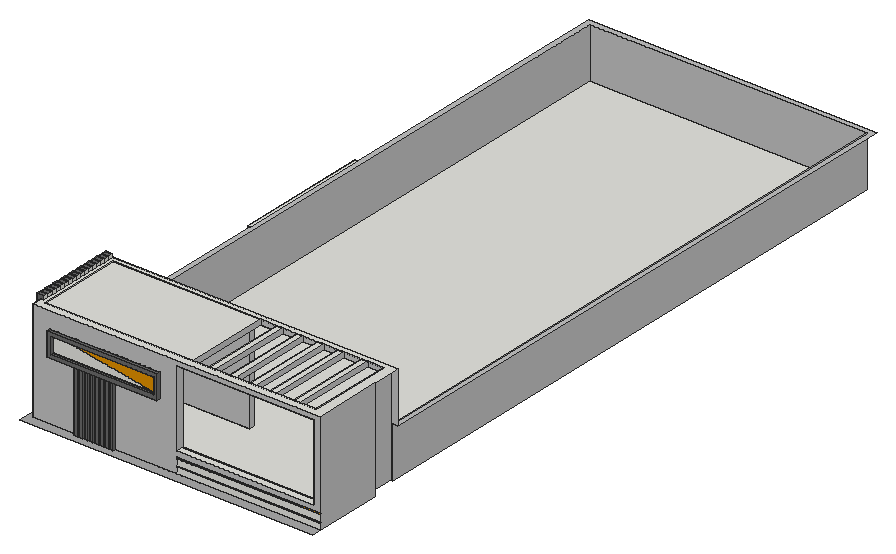
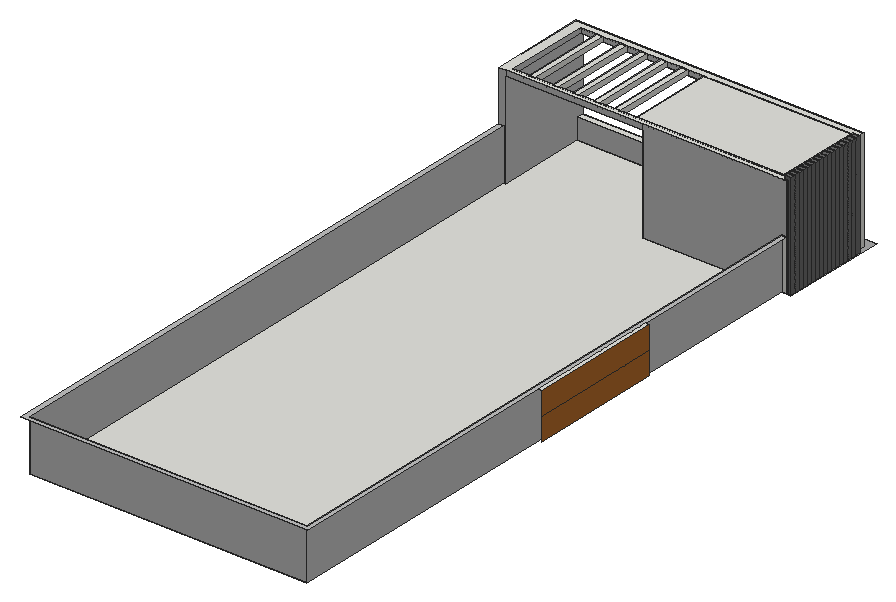
# SketchUp Ruby script. Lengths in inches.
U = 1.inch
M = Sketchup.active_model
def pt(a) = Geom::Point3d.new(a.map { |v| v * U })
def face(e, loops, mat)
  f = e.add_face(loops[0].map { |a| pt(a) })
  loops[1..].each { |l| e.add_face(l.map { |a| pt(a) }).erase! }
  f.material = f.back_material = mat if mat
  f
end
# faces: each face lists its corners as indices into pts; further lists are holes
def faces(e, pts, list, mat = nil) = list.each { |f| face(e, (f[0].is_a?(Array) ? f : [f]).map { |l| l.map { |i| pts[i] } }, mat) }
# xy, xz, yz: faces in a plane at the given z, y or x. An outline is a flat list of corners, or four numbers for a rectangle; further outlines are holes
def ring(l) = l.size == 4 ? [[l[0], l[1]], [l[2], l[1]], [l[2], l[3]], [l[0], l[3]]] : l.each_slice(2).to_a
def flat(e, list, mat, &to3) = list.each { |f| face(e, (f[0].is_a?(Array) ? f : [f]).map { |l| ring(l).map { |u, v| to3.(u, v) } }, mat) }
def xy(e, z, list, mat = nil) = flat(e, list, mat) { |x, y| [x, y, z] }
def xz(e, y, list, mat = nil) = flat(e, list, mat) { |x, z| [x, y, z] }
def yz(e, x, list, mat = nil) = flat(e, list, mat) { |y, z| [x, y, z] }
def lines(e, pts, list) = list.each { |a, b| e.add_line(pt(pts[a]), pt(pts[b])) }
# prism: a flat outline (further loops are holes) pulled along v
def prism(e, loops, v, mat = nil)
  f = face(e, loops, mat); d = Geom::Vector3d.new(v.map { |x| x * U })
  f.pushpull(f.normal.samedirection?(d) ? d.length : -d.length)
end
def box(e, o, s, mat = nil) = prism(e, [[o, [o[0] + s[0], o[1], o[2]], [o[0] + s[0], o[1] + s[1], o[2]], [o[0], o[1] + s[1], o[2]]]], [0, 0, s[2]], mat)
def at(x, y, z, deg = 0) = Geom::Transformation.translation(pt([x, y, z])) * Geom::Transformation.rotation(ORIGIN, Z_AXIS, deg.degrees)
def axes(o, x, y, z) = Geom::Transformation.new([*x, 0, *y, 0, *z, 0, *pt(o).to_a, 1])
def part(name) = M.definitions.add(name)
# library, detail: a bought-in or finely detailed component or shape, given as its bounding box
def library(name, o, s) = part(name).tap { |d| box(d.entities, o, s) }
def detail(e, o, s) = box(e.add_group.entities, o, s)
def put(e, d, t, mat = nil) = e.add_instance(d, t).tap { |i| i.material = mat if mat }
def group(e, t, mat = nil) = e.add_group.tap { |g| g.transformation = t; g.material = mat if mat }.entities
root = M.entities
M.materials.add("[0038_Orange]").color = [221, 143, 0]
M.materials.add("[0131_Silver]").color = [192, 192, 192]
M.materials.add("[0132_LightGray]").color = [169, 169, 169]
M.materials.add("[0134_DimGray]").color = [105, 105, 105]
M.materials.add("[Wood Bamboo]").color = [177, 105, 43]
xy(root,996,[[72,36,72,378,582,378,582,360,96,360,96,60,582,60,582,36],[582,36,1068,60],[96,60,1068,60,1068,378,1074,378,1074,2478,90,2478,90,378,582,378,582,360,96,360],[57.95,71.51,70.26,86.51],[57.95,89.51,70.26,104.51],
  [57.95,107.51,70.26,122.51],[57.95,125.51,70.26,140.51],[57.95,143.51,70.26,158.51],[57.95,161.51,70.26,176.51],[57.95,179.51,70.26,194.51],
  [57.95,197.51,70.26,212.51],[57.95,215.51,70.26,230.51],[57.95,233.51,70.26,248.51],[57.95,251.51,70.26,266.51],[57.95,269.51,70.26,284.51],
  [57.95,287.51,70.26,302.51],[57.95,305.51,70.26,320.51],[57.95,323.51,70.26,338.51],[57.95,341.51,70.26,356.51],[57.95,359.51,70.26,374.51]])
xy(root,996,[[[56,0,1092,0,1092,36,72,36,72,378,56,378],[57.95,359.51,70.26,374.51],[57.95,341.51,70.26,356.51],[57.95,323.51,70.26,338.51],[57.95,305.51,70.26,320.51],[57.95,287.51,70.26,302.51],[57.95,269.51,70.26,284.51],[57.95,251.51,70.26,266.51],[57.95,233.51,70.26,248.51],[57.95,215.51,70.26,230.51],[57.95,197.51,70.26,212.51],[57.95,179.51,70.26,194.51],[57.95,161.51,70.26,176.51],[57.95,143.51,70.26,158.51],[57.95,125.51,70.26,140.51],[57.95,107.51,70.26,122.51],[57.95,89.51,70.26,104.51],[57.95,71.51,70.26,86.51],[261.49,26.61,275.24,33.55],[225.49,26.61,239.24,33.55],[315.49,26.61,329.24,33.55],[243.49,26.61,257.24,33.55],[279.49,26.61,293.24,33.55],[297.49,26.61,311.24,33.55],[333.49,26.61,347.24,33.55],[351.22,26.61,362.44,33.55]]],"[0132_LightGray]")
xy(root,1015.2,[[582,36,1092,39]],"[0038_Orange]")
xy(root,1021.2,[[582,36,1092,39]],"[0038_Orange]")
xy(root,1042.8,[[582,36,1092,39]],"[0038_Orange]")
xy(root,1048.8,[[582,36,1092,39]],"[0038_Orange]")
xy(root,1068,[[582,36,1068,60]])
xy(root,1176,[[60,1000.8,72,1476]])
xy(root,1176,[[72,378,90,378,90,2478,1074,2478,1074,378,1092,378,1092,2496,72,2496]],"[0131_Silver]")
xy(root,1212,[[225.49,26.61,239.24,33.55],[243.49,26.61,257.24,33.55],[261.49,26.61,275.24,33.55],[279.49,26.61,293.24,33.55],[297.49,26.61,311.24,33.55],
  [315.49,26.61,329.24,33.55],[333.49,26.61,347.24,33.55],[351.22,26.61,362.44,33.55]])
xy(root,1212,[[[132,23,522,36],[225.49,26.61,239.24,33.55],[243.49,26.61,257.24,33.55],[261.49,26.61,275.24,33.55],[279.49,26.61,293.24,33.55],[297.49,26.61,311.24,33.55],[315.49,26.61,329.24,33.55],[333.49,26.61,347.24,33.55],[351.22,26.61,362.44,33.55]]],"[0134_DimGray]")
xy(root,1224,[[144,23,510,36]],"[0134_DimGray]")
xy(root,1284,[[144,23,510,36]],"[0134_DimGray]")
xy(root,1296,[[132,23,522,36]],"[0134_DimGray]")
xy(root,1338,[[688.58,169.22,687.03,169.43,685.58,170.03,684.34,170.98,683.39,172.22,682.79,173.67,682.58,175.22,682.79,176.78,683.39,178.22,684.34,179.47,685.58,180.42,687.03,181.02,688.58,181.22,690.14,181.02,691.58,180.42,692.83,179.47,693.78,178.22,694.38,176.78,694.58,175.22,694.38,173.67,693.78,172.22,692.83,170.98,691.58,170.03,690.14,169.43],[758.83,169.22,757.28,169.43,755.83,170.03,754.59,170.98,753.64,172.22,753.04,173.67,752.83,175.22,753.04,176.78,753.64,178.22,754.59,179.47,755.83,180.42,757.28,181.02,758.83,181.22,760.39,181.02,761.83,180.42,763.08,179.47,764.03,178.22,764.63,176.78,764.83,175.22,764.63,173.67,764.03,172.22,763.08,170.98,761.83,170.03,760.39,169.43],[832.15,169.22,830.59,169.43,829.15,170.03,827.9,170.98,826.95,172.22,826.35,173.67,826.15,175.22,826.35,176.78,826.95,178.22,827.9,179.47,829.15,180.42,830.59,181.02,832.15,181.22,833.7,181.02,835.15,180.42,836.39,179.47,837.34,178.22,837.94,176.78,838.15,175.22,837.94,173.67,837.34,172.22,836.39,170.98,835.15,170.03,833.7,169.43],[903.27,169.22,901.72,169.43,900.27,170.03,899.03,170.98,898.07,172.22,897.47,173.67,897.27,175.22,897.47,176.78,898.07,178.22,899.03,179.47,900.27,180.42,901.72,181.02,903.27,181.22,904.82,181.02,906.27,180.42,907.51,179.47,908.47,178.22,909.07,176.78,909.27,175.22,909.07,173.67,908.47,172.22,907.51,170.98,906.27,170.03,904.82,169.43],[987.4,169.22,985.84,169.43,984.4,170.03,983.15,170.98,982.2,172.22,981.6,173.67,981.4,175.22,981.6,176.78,982.2,178.22,983.15,179.47,984.4,180.42,985.84,181.02,987.4,181.22,988.95,181.02,990.4,180.42,991.64,179.47,992.59,178.22,993.19,176.78,993.4,175.22,993.19,173.67,992.59,172.22,991.64,170.98,990.4,170.03,988.95,169.43]])
xy(root,1338,[[582,36,582,60,1056,60,1056,360,582,360,582,378,1068,378,1068,36],[96,60,619.28,360],[[676.64,60,698.28,360],[688.58,169.22,690.14,169.43,691.58,170.03,692.83,170.98,693.78,172.22,694.38,173.67,694.58,175.22,694.38,176.78,693.78,178.22,692.83,179.47,691.58,180.42,690.14,181.02,688.58,181.22,687.03,181.02,685.58,180.42,684.34,179.47,683.39,178.22,682.79,176.78,682.58,175.22,682.79,173.67,683.39,172.22,684.34,170.98,685.58,170.03,687.03,169.43]],[[748.64,60,770.28,360],[758.83,169.22,760.39,169.43,761.83,170.03,763.08,170.98,764.03,172.22,764.63,173.67,764.83,175.22,764.63,176.78,764.03,178.22,763.08,179.47,761.83,180.42,760.39,181.02,758.83,181.22,757.28,181.02,755.83,180.42,754.59,179.47,753.64,178.22,753.04,176.78,752.83,175.22,753.04,173.67,753.64,172.22,754.59,170.98,755.83,170.03,757.28,169.43]],[[820.64,60,842.28,360],[832.15,169.22,833.7,169.43,835.15,170.03,836.39,170.98,837.34,172.22,837.94,173.67,838.15,175.22,837.94,176.78,837.34,178.22,836.39,179.47,835.15,180.42,833.7,181.02,832.15,181.22,830.59,181.02,829.15,180.42,827.9,179.47,826.95,178.22,826.35,176.78,826.15,175.22,826.35,173.67,826.95,172.22,827.9,170.98,829.15,170.03,830.59,169.43]],
  [[892.64,60,914.28,360],[903.27,169.22,904.82,169.43,906.27,170.03,907.51,170.98,908.47,172.22,909.07,173.67,909.27,175.22,909.07,176.78,908.47,178.22,907.51,179.47,906.27,180.42,904.82,181.02,903.27,181.22,901.72,181.02,900.27,180.42,899.03,179.47,898.07,178.22,897.47,176.78,897.27,175.22,897.47,173.67,898.07,172.22,899.03,170.98,900.27,170.03,901.72,169.43]],[[976.64,60,998.28,360],[987.4,169.22,988.95,169.43,990.4,170.03,991.64,170.98,992.59,172.22,993.19,173.67,993.4,175.22,993.19,176.78,992.59,178.22,991.64,179.47,990.4,180.42,988.95,181.02,987.4,181.22,985.84,181.02,984.4,180.42,983.15,179.47,982.2,178.22,981.6,176.78,981.4,175.22,981.6,173.67,982.2,172.22,983.15,170.98,984.4,170.03,985.84,169.43]]],"[0131_Silver]")
xy(root,1356,[[[72,36,1092,36,1092,378,72,378,72,374.51,82.26,374.51,82.26,359.51,72,359.51,72,356.51,82.26,356.51,82.26,341.51,72,341.51,72,338.51,82.26,338.51,82.26,323.51,72,323.51,72,320.51,82.26,320.51,82.26,305.51,72,305.51,72,302.51,82.26,302.51,82.26,287.51,72,287.51,72,284.51,82.26,284.51,82.26,269.51,72,269.51,72,266.51,82.26,266.51,82.26,251.51,72,251.51,72,248.51,82.26,248.51,82.26,233.51,72,233.51,72,230.51,82.26,230.51,82.26,215.51,72,215.51,72,212.51,82.26,212.51,82.26,197.51,72,197.51,72,194.51,82.26,194.51,82.26,179.51,72,179.51,72,176.51,82.26,176.51,82.26,161.51,72,161.51,72,158.51,82.26,158.51,82.26,143.51,72,143.51,72,140.51,82.26,140.51,82.26,125.51,72,125.51,72,122.51,82.26,122.51,82.26,107.51,72,107.51,72,104.51,82.26,104.51,82.26,89.51,72,89.51,72,86.51,82.26,86.51,82.26,71.51,72,71.51],[96,60,1056,360]],[96,60,619.28,360],[676.64,60,698.28,360],[748.64,60,770.28,360],[820.64,60,842.28,360],
  [892.64,60,914.28,360],[976.64,60,998.28,360],[70.26,71.51,72,86.51],[72,71.51,82.26,86.51],[70.26,89.51,72,104.51],
  [72,89.51,82.26,104.51],[70.26,107.51,72,122.51],[72,107.51,82.26,122.51],[70.26,125.51,72,140.51],[72,125.51,82.26,140.51],
  [70.26,143.51,72,158.51],[72,143.51,82.26,158.51],[70.26,161.51,72,176.51],[72,161.51,82.26,176.51],[70.26,179.51,72,194.51],
  [72,179.51,82.26,194.51],[70.26,197.51,72,212.51],[72,197.51,82.26,212.51],[70.26,215.51,72,230.51],[72,215.51,82.26,230.51],
  [70.26,233.51,72,248.51],[72,233.51,82.26,248.51],[70.26,251.51,72,266.51],[72,251.51,82.26,266.51],[70.26,269.51,72,284.51],
  [72,269.51,82.26,284.51],[70.26,287.51,72,302.51],[72,287.51,82.26,302.51],[70.26,305.51,72,320.51],[72,305.51,82.26,320.51],
  [70.26,323.51,72,338.51],[72,323.51,82.26,338.51],[70.26,341.51,72,356.51],[72,341.51,82.26,356.51],[70.26,359.51,72,374.51],
  [72,359.51,82.26,374.51]])
xy(root,1368,[[57.95,71.51,82.26,86.51],[57.95,89.51,82.26,104.51],[57.95,107.51,82.26,122.51],[57.95,125.51,82.26,140.51],[57.95,143.51,82.26,158.51],
  [57.95,161.51,82.26,176.51],[57.95,179.51,82.26,194.51],[57.95,197.51,82.26,212.51],[57.95,215.51,82.26,230.51],[57.95,233.51,82.26,248.51],
  [57.95,251.51,82.26,266.51],[57.95,269.51,82.26,284.51],[57.95,287.51,82.26,302.51],[57.95,305.51,82.26,320.51],[57.95,323.51,82.26,338.51],
  [57.95,341.51,82.26,356.51],[57.95,359.51,82.26,374.51]],"[0134_DimGray]")
xz(root,23,[[[132,1212,522,1296],[144,1224,510,1284]]],"[0134_DimGray]")
xz(root,26.61,[[225.49,996,239.24,1212],[243.49,996,257.24,1212],[261.49,996,275.24,1212],[279.49,996,293.24,1212],[297.49,996,311.24,1212],
  [315.49,996,329.24,1212],[333.49,996,347.24,1212],[351.22,996,362.44,1212]],"[0134_DimGray]")
xz(root,33.55,[[225.49,996,239.24,1212],[243.49,996,257.24,1212],[261.49,996,275.24,1212],[279.49,996,293.24,1212],[297.49,996,311.24,1212],
  [315.49,996,329.24,1212],[333.49,996,347.24,1212],[351.22,996,362.44,1212]])
xz(root,36,[[582,996,1092,1015.2],[582,1021.2,1092,1042.8],[[132,1212,522,1296],[144,1224,510,1284]],[144,1224,510,1224,144,1284]])
xz(root,36,[[510,1224,510,1284,144,1284]],"[0038_Orange]")
xz(root,36,[[[72,996,582,996,582,1338,1068,1338,1068,1068,582,1068,582,1048.8,1092,1048.8,1092,1356,72,1356],[132,1212,522,1296]]],"[0131_Silver]")
xz(root,39,[[582,1015.2,1092,1021.2],[582,1042.8,1092,1048.8]],"[0038_Orange]")
xz(root,60,[[96,1338,582,1356],[582,1338,604.64,1356],[604.64,1338,619.28,1356],[676.64,1338,691.28,1356],[691.28,1338,698.28,1356],
  [748.64,1338,763.28,1356],[763.28,1338,770.28,1356],[820.64,1338,835.28,1356],[835.28,1338,842.28,1356],[892.64,1338,907.28,1356],
  [907.28,1338,914.28,1356],[976.64,1338,991.28,1356],[991.28,1338,998.28,1356]])
xz(root,60,[[96,996,96,1338,582,1338,582,1068,1068,1068,1068,996],[619.28,1338,676.64,1356],[698.28,1338,748.64,1356],[770.28,1338,820.64,1356],[842.28,1338,892.64,1356],
  [914.28,1338,976.64,1356],[998.28,1338,1056,1356]],"[0131_Silver]")
xz(root,71.51,[[57.95,996,70.26,996,70.26,1356,82.26,1356,82.26,1368,57.95,1368]],"[0134_DimGray]")
xz(root,86.51,[[57.95,996,57.95,1368,82.26,1368,82.26,1356,70.26,1356,70.26,996]],"[0134_DimGray]")
xz(root,89.51,[[57.95,996,70.26,996,70.26,1356,82.26,1356,82.26,1368,57.95,1368]],"[0134_DimGray]")
xz(root,104.51,[[57.95,996,57.95,1368,82.26,1368,82.26,1356,70.26,1356,70.26,996]],"[0134_DimGray]")
xz(root,107.51,[[57.95,996,70.26,996,70.26,1356,82.26,1356,82.26,1368,57.95,1368]],"[0134_DimGray]")
xz(root,122.51,[[57.95,996,57.95,1368,82.26,1368,82.26,1356,70.26,1356,70.26,996]],"[0134_DimGray]")
xz(root,125.51,[[57.95,996,70.26,996,70.26,1356,82.26,1356,82.26,1368,57.95,1368]],"[0134_DimGray]")
xz(root,140.51,[[57.95,996,57.95,1368,82.26,1368,82.26,1356,70.26,1356,70.26,996]],"[0134_DimGray]")
xz(root,143.51,[[57.95,996,70.26,996,70.26,1356,82.26,1356,82.26,1368,57.95,1368]],"[0134_DimGray]")
xz(root,158.51,[[57.95,996,57.95,1368,82.26,1368,82.26,1356,70.26,1356,70.26,996]],"[0134_DimGray]")
xz(root,161.51,[[57.95,996,70.26,996,70.26,1356,82.26,1356,82.26,1368,57.95,1368]],"[0134_DimGray]")
xz(root,176.51,[[57.95,996,57.95,1368,82.26,1368,82.26,1356,70.26,1356,70.26,996]],"[0134_DimGray]")
xz(root,179.51,[[57.95,996,70.26,996,70.26,1356,82.26,1356,82.26,1368,57.95,1368]],"[0134_DimGray]")
xz(root,194.51,[[57.95,996,57.95,1368,82.26,1368,82.26,1356,70.26,1356,70.26,996]],"[0134_DimGray]")
xz(root,197.51,[[57.95,996,70.26,996,70.26,1356,82.26,1356,82.26,1368,57.95,1368]],"[0134_DimGray]")
xz(root,212.51,[[57.95,996,57.95,1368,82.26,1368,82.26,1356,70.26,1356,70.26,996]],"[0134_DimGray]")
xz(root,215.51,[[57.95,996,70.26,996,70.26,1356,82.26,1356,82.26,1368,57.95,1368]],"[0134_DimGray]")
xz(root,230.51,[[57.95,996,57.95,1368,82.26,1368,82.26,1356,70.26,1356,70.26,996]],"[0134_DimGray]")
xz(root,233.51,[[57.95,996,70.26,996,70.26,1356,82.26,1356,82.26,1368,57.95,1368]],"[0134_DimGray]")
xz(root,248.51,[[57.95,996,57.95,1368,82.26,1368,82.26,1356,70.26,1356,70.26,996]],"[0134_DimGray]")
xz(root,251.51,[[57.95,996,70.26,996,70.26,1356,82.26,1356,82.26,1368,57.95,1368]],"[0134_DimGray]")
xz(root,266.51,[[57.95,996,57.95,1368,82.26,1368,82.26,1356,70.26,1356,70.26,996]],"[0134_DimGray]")
xz(root,269.51,[[57.95,996,70.26,996,70.26,1356,82.26,1356,82.26,1368,57.95,1368]],"[0134_DimGray]")
xz(root,284.51,[[57.95,996,57.95,1368,82.26,1368,82.26,1356,70.26,1356,70.26,996]],"[0134_DimGray]")
xz(root,287.51,[[57.95,996,70.26,996,70.26,1356,82.26,1356,82.26,1368,57.95,1368]],"[0134_DimGray]")
xz(root,302.51,[[57.95,996,57.95,1368,82.26,1368,82.26,1356,70.26,1356,70.26,996]],"[0134_DimGray]")
xz(root,305.51,[[57.95,996,70.26,996,70.26,1356,82.26,1356,82.26,1368,57.95,1368]],"[0134_DimGray]")
xz(root,320.51,[[57.95,996,57.95,1368,82.26,1368,82.26,1356,70.26,1356,70.26,996]],"[0134_DimGray]")
xz(root,323.51,[[57.95,996,70.26,996,70.26,1356,82.26,1356,82.26,1368,57.95,1368]],"[0134_DimGray]")
xz(root,338.51,[[57.95,996,57.95,1368,82.26,1368,82.26,1356,70.26,1356,70.26,996]],"[0134_DimGray]")
xz(root,341.51,[[57.95,996,70.26,996,70.26,1356,82.26,1356,82.26,1368,57.95,1368]],"[0134_DimGray]")
xz(root,356.51,[[57.95,996,57.95,1368,82.26,1368,82.26,1356,70.26,1356,70.26,996]],"[0134_DimGray]")
xz(root,359.51,[[57.95,996,70.26,996,70.26,1356,82.26,1356,82.26,1368,57.95,1368]],"[0134_DimGray]")
xz(root,360,[[96,1338,582,1356],[582,1338,604.64,1356],[604.64,1338,619.28,1356],[676.64,1338,691.28,1356],[691.28,1338,698.28,1356],
  [748.64,1338,763.28,1356],[763.28,1338,770.28,1356],[820.64,1338,835.28,1356],[835.28,1338,842.28,1356],[892.64,1338,907.28,1356],
  [907.28,1338,914.28,1356],[976.64,1338,991.28,1356],[991.28,1338,998.28,1356]])
xz(root,360,[[96,996,582,1338],[619.28,1338,676.64,1356],[698.28,1338,748.64,1356],[770.28,1338,820.64,1356],[842.28,1338,892.64,1356],
  [914.28,1338,976.64,1356],[998.28,1338,1056,1356]],"[0131_Silver]")
xz(root,374.51,[[57.95,996,57.95,1368,82.26,1368,82.26,1356,70.26,1356,70.26,996]],"[0134_DimGray]")
xz(root,378,[[72,996,90,1176]])
xz(root,378,[[90,996,90,1176,72,1176,72,1356,582,1356,582,996],[1068,996,1068,1356,1092,1356,1092,1176,1074,1176,1074,996],[582,1338,1068,1356]],"[0131_Silver]")
xz(root,2478,[[90,996,1074,1176]],"[0131_Silver]")
yz(root,57.95,[[71.51,996,86.51,1368],[89.51,996,104.51,1368],[107.51,996,122.51,1368],[125.51,996,140.51,1368],[143.51,996,158.51,1368],
  [161.51,996,176.51,1368],[179.51,996,194.51,1368],[197.51,996,212.51,1368],[215.51,996,230.51,1368],[233.51,996,248.51,1368],
  [251.51,996,266.51,1368],[269.51,996,284.51,1368],[287.51,996,302.51,1368],[305.51,996,320.51,1368],[323.51,996,338.51,1368],
  [341.51,996,356.51,1368],[359.51,996,374.51,1368]],"[0134_DimGray]")
yz(root,60,[[1000.8,1014,1476,1092],[1000.8,1092,1476,1176]],"[Wood Bamboo]")
yz(root,70.26,[[71.51,996,86.51,1356],[89.51,996,104.51,1356],[107.51,996,122.51,1356],[125.51,996,140.51,1344.8125],[143.51,996,158.51,1348.1875],
  [161.51,996,176.51,1356],[179.51,996,194.51,1356],[197.51,996,212.51,1356],[215.51,996,230.51,1032],[233.51,996,248.51,1356],
  [251.51,996,266.51,1356],[269.51,996,284.51,1356],[287.51,996,302.51,1356],[305.51,996,320.51,1356],[323.51,996,338.51,1356],
  [341.51,996,356.51,1356],[359.51,996,374.51,1356],[215.51,1032,230.51,1356],[125.51,1344.8125,140.51,1356],[143.51,1348.1875,158.51,1356]])
yz(root,72,[[36,996,378,1356]])
yz(root,82.26,[[71.51,1356,86.51,1368],[89.51,1356,104.51,1368],[107.51,1356,122.51,1368],[125.51,1356,140.51,1368],[143.51,1356,158.51,1368],
  [161.51,1356,176.51,1368],[179.51,1356,194.51,1368],[197.51,1356,212.51,1368],[215.51,1356,230.51,1368],[233.51,1356,248.51,1368],
  [251.51,1356,266.51,1368],[269.51,1356,284.51,1368],[287.51,1356,302.51,1368],[305.51,1356,320.51,1368],[323.51,1356,338.51,1368],
  [341.51,1356,356.51,1368],[359.51,1356,374.51,1368]])
yz(root,90,[[378,996,2478,1176]],"[0131_Silver]")
yz(root,96,[[60,1338,360,1356]])
yz(root,96,[[60,996,360,1338]],"[0131_Silver]")
yz(root,132,[[23,1212,36,1296]],"[0134_DimGray]")
yz(root,144,[[23,1224,36,1284]],"[0134_DimGray]")
yz(root,225.49,[[26.61,996,33.55,1212]],"[0134_DimGray]")
yz(root,239.24,[[26.61,996,33.55,1212]],"[0134_DimGray]")
yz(root,243.49,[[26.61,996,33.55,1212]],"[0134_DimGray]")
yz(root,257.24,[[26.61,996,33.55,1212]],"[0134_DimGray]")
yz(root,261.49,[[26.61,996,33.55,1212]],"[0134_DimGray]")
yz(root,275.24,[[26.61,996,33.55,1212]],"[0134_DimGray]")
yz(root,279.49,[[26.61,996,33.55,1212]],"[0134_DimGray]")
yz(root,293.24,[[26.61,996,33.55,1212]],"[0134_DimGray]")
yz(root,297.49,[[26.61,996,33.55,1212]],"[0134_DimGray]")
yz(root,311.24,[[26.61,996,33.55,1212]],"[0134_DimGray]")
yz(root,315.49,[[26.61,996,33.55,1212]],"[0134_DimGray]")
yz(root,329.24,[[26.61,996,33.55,1212]],"[0134_DimGray]")
yz(root,333.49,[[26.61,996,33.55,1212]],"[0134_DimGray]")
yz(root,347.24,[[26.61,996,33.55,1212]],"[0134_DimGray]")
yz(root,351.22,[[26.61,996,33.55,1212]],"[0134_DimGray]")
yz(root,362.44,[[26.61,996,33.55,1212]],"[0134_DimGray]")
yz(root,510,[[23,1224,36,1284]],"[0134_DimGray]")
yz(root,522,[[23,1212,36,1296]],"[0134_DimGray]")
yz(root,582,[[36,1015.2,39,1021.2],[36,1042.8,39,1048.8]],"[0038_Orange]")
yz(root,582,[[360,996,378,1338],[36,1068,60,1338]],"[0131_Silver]")
yz(root,619.28,[[60,1338,360,1356]],"[0131_Silver]")
yz(root,676.64,[[60,1338,360,1356]])
yz(root,698.28,[[60,1338,360,1356]],"[0131_Silver]")
yz(root,748.64,[[60,1338,360,1356]])
yz(root,770.28,[[60,1338,360,1356]],"[0131_Silver]")
yz(root,820.64,[[60,1338,360,1356]])
yz(root,842.28,[[60,1338,360,1356]],"[0131_Silver]")
yz(root,892.64,[[60,1338,360,1356]])
yz(root,914.28,[[60,1338,360,1356]],"[0131_Silver]")
yz(root,976.64,[[60,1338,360,1356]])
yz(root,998.28,[[60,1338,360,1356]],"[0131_Silver]")
yz(root,1056,[[60,1338,360,1356]],"[0131_Silver]")
yz(root,1068,[[60,996,60,1068,36,1068,36,1338,378,1338,378,996]],"[0131_Silver]")
yz(root,1074,[[378,996,2478,1176]],"[0131_Silver]")
yz(root,1092,[[36,996,276,996,276,1356,36,1356,36,1048.8,39,1048.8,39,1042.8,36,1042.8,36,1021.2,39,1021.2,39,1015.2,36,1015.2]],"[0131_Silver]")
p = [[1074,378,996],[1092,378,996],[1068,360,1338],[1068,360,1356]]
lines(root,p,[[0,1],[2,3]])
